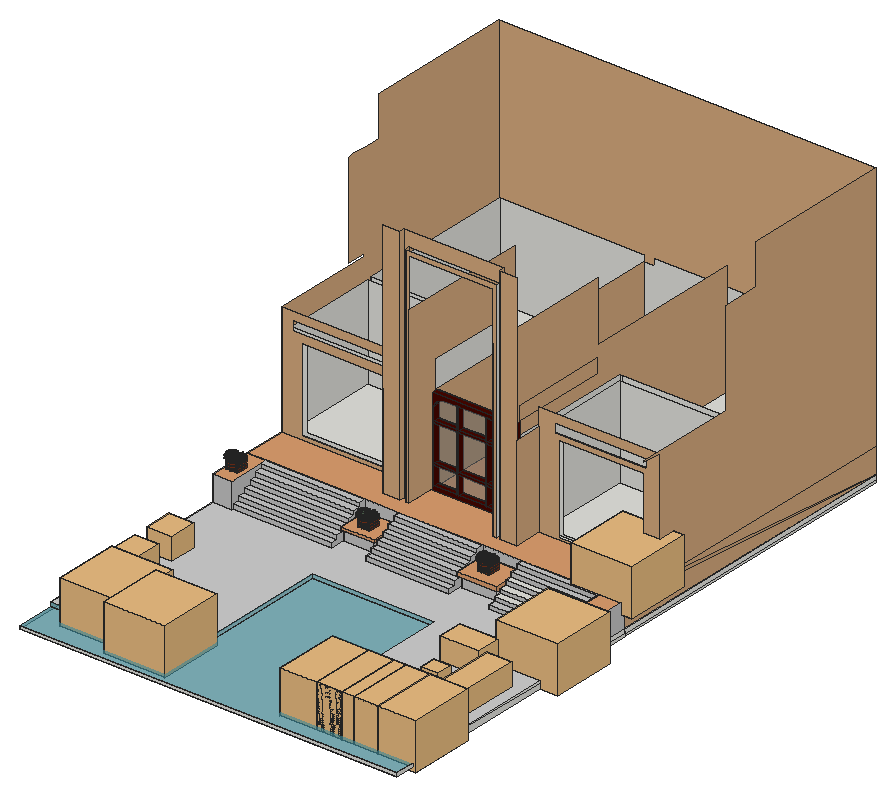
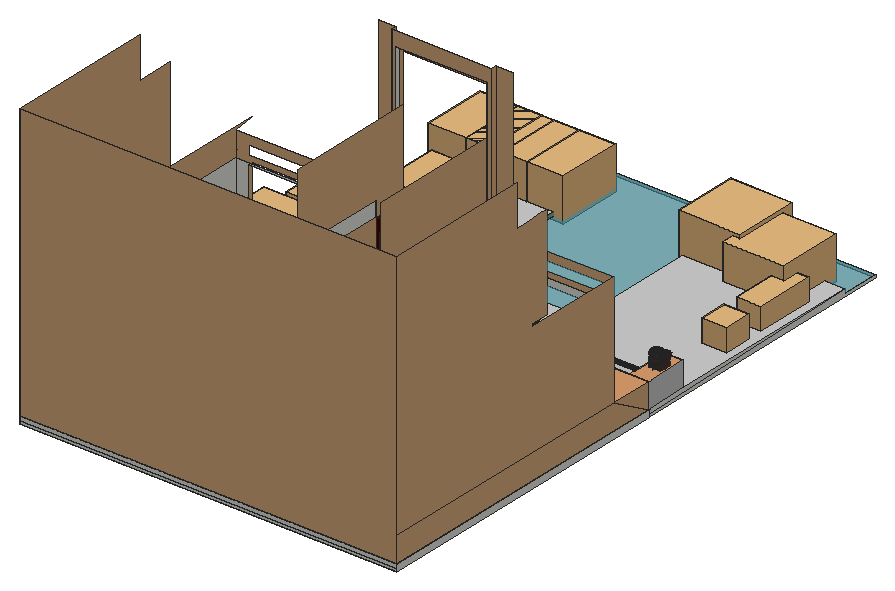
# SketchUp Ruby script. Lengths in inches.
U = 1.inch
M = Sketchup.active_model
def pt(a) = Geom::Point3d.new(a.map { |v| v * U })
def face(e, loops, mat)
  f = e.add_face(loops[0].map { |a| pt(a) })
  loops[1..].each { |l| e.add_face(l.map { |a| pt(a) }).erase! }
  f.material = f.back_material = mat if mat
  f
end
# faces: each face lists its corners as indices into pts; further lists are holes
def faces(e, pts, list, mat = nil) = list.each { |f| face(e, (f[0].is_a?(Array) ? f : [f]).map { |l| l.map { |i| pts[i] } }, mat) }
# xy, xz, yz: faces in a plane at the given z, y or x. An outline is a flat list of corners, or four numbers for a rectangle; further outlines are holes
def ring(l) = l.size == 4 ? [[l[0], l[1]], [l[2], l[1]], [l[2], l[3]], [l[0], l[3]]] : l.each_slice(2).to_a
def flat(e, list, mat, &to3) = list.each { |f| face(e, (f[0].is_a?(Array) ? f : [f]).map { |l| ring(l).map { |u, v| to3.(u, v) } }, mat) }
def xy(e, z, list, mat = nil) = flat(e, list, mat) { |x, y| [x, y, z] }
def xz(e, y, list, mat = nil) = flat(e, list, mat) { |x, z| [x, y, z] }
def yz(e, x, list, mat = nil) = flat(e, list, mat) { |y, z| [x, y, z] }
def lines(e, pts, list) = list.each { |a, b| e.add_line(pt(pts[a]), pt(pts[b])) }
# prism: a flat outline (further loops are holes) pulled along v
def prism(e, loops, v, mat = nil)
  f = face(e, loops, mat); d = Geom::Vector3d.new(v.map { |x| x * U })
  f.pushpull(f.normal.samedirection?(d) ? d.length : -d.length)
end
def box(e, o, s, mat = nil) = prism(e, [[o, [o[0] + s[0], o[1], o[2]], [o[0] + s[0], o[1] + s[1], o[2]], [o[0], o[1] + s[1], o[2]]]], [0, 0, s[2]], mat)
def at(x, y, z, deg = 0) = Geom::Transformation.translation(pt([x, y, z])) * Geom::Transformation.rotation(ORIGIN, Z_AXIS, deg.degrees)
def axes(o, x, y, z) = Geom::Transformation.new([*x, 0, *y, 0, *z, 0, *pt(o).to_a, 1])
def part(name) = M.definitions.add(name)
# library, detail: a bought-in or finely detailed component or shape, given as its bounding box
def library(name, o, s) = part(name).tap { |d| box(d.entities, o, s) }
def detail(e, o, s) = box(e.add_group.entities, o, s)
def put(e, d, t, mat = nil) = e.add_instance(d, t).tap { |i| i.material = mat if mat }
def group(e, t, mat = nil) = e.add_group.tap { |g| g.transformation = t; g.material = mat if mat }.entities
root = M.entities
M.materials.add("24").color = [120, 49, 24]
M.materials.add("[Carrera Marble]").color = [207, 207, 207]
M.materials.add("[Color C04]").color = [215, 171, 127]
M.materials.add("[Color C04]1").color = [220, 158, 110]
M.materials.add("[Color C08]").color = [71, 7, 0]
M.materials.add("[Color M02]").color = [198, 198, 198]
M.materials.add("[Color_G20]").color = [81, 102, 81]
M.materials.add("[Translucent Glass Gray]").color = [128, 128, 128]
M.materials["[Translucent Glass Gray]"].alpha = 0.5
M.materials.add("[Water Pool Light]").color = [64, 149, 167]
M.materials["[Water Pool Light]"].alpha = 0.6
c1 = library("VASO",[-61.49,-57.125,-14.62],[117.55,124.5,88.55])
c2 = library("Group\#4",[0,0,0],[47.0625,53.38,42.38])
c3 = part("3 Leaves\#1")
g1 = group(c3.entities,at(19.98,16.45,10.46))
p = [[9.41,-13.74,-5.37],[9.39,-13.76,-5.36],[9.41,-13.74,-5.375],[-2.22,-4.52,-2],[-1.83,-5.58,-2.64],[-1.27,-6.61,-3.21],
  [-0.57,-7.58,-3.71],[0.27,-8.49,-4.12],[1.23,-9.31,-4.4375],[2.29,-10.02,-4.66],[3.44,-10.62,-4.77],[4.65,-11.09,-4.78],
  [5.91,-11.43,-4.6875],[7.18,-11.625,-4.49],[-2.5,-2.36,-0.58],[-2.44,-3.4375,-1.3125],[0.95,-3.95,0.875],[-0.22,-3.3,0.57],
  [-1.375,-2.77,0.09],[7.11,-10.89,-3.34],[6.85,-10.07,-2.28],[6.41,-9.18,-1.33],[5.81,-8.27,-0.52],[5.05,-7.33,0.125],
  [4.16,-6.41,0.6],[3.16,-5.53,0.89],[2.08,-4.7,0.98],[7.17,-11.64,-4.47],[7.19,-11.61,-4.47]]
faces(g1,p,[[0,1,2],[13,27,28]])
faces(g1,p,[[3,4,5,6,7,8,9,10,11,12,13,14,15],[16,17,18,14,13,19,20,21,22,23,24,25,26]],"[Color_G20]")
g2 = group(c3.entities,at(13.74,14.6,8.97))
p = [[1.36,-2.61,0.95],[2.62,-2.08,0.98],[-2.43,-12.26,-7.12],[-3.0625,-11.53,-6.15],[-3.5,-10.7,-5.16],[-3.74,-9.79,-4.17],
  [-3.77,-8.82,-3.21],[-3.58,-7.83,-2.29],[-3.18,-6.82,-1.46],[-2.59,-5.84,-0.71],[-1.82,-4.91,-0.09],[-0.89,-4.04,0.4],
  [0.18,-3.27,0.75],[-2.43,-12.27,-7.1],[-2.45,-12.25,-7.12],[3.08,-3.14,0.39],[3.37,-4.23,-0.27],[3.49,-5.32,-0.97],
  [3.44,-6.39,-1.7],[3.22,-7.43,-2.45],[2.83,-8.42,-3.21],[2.28,-9.33,-3.96],[1.58,-10.15,-4.68],[0.74,-10.86,-5.375],
  [-0.22,-11.46,-6.02],[-1.28,-11.93,-6.6]]
faces(g2,p,[[0,1,2,3,4,5,6,7,8,9,10,11,12],[2,1,15,16,17,18,19,20,21,22,23,24,25]],"[Color_G20]")
faces(g2,p,[[2,13,14]])
g3 = group(c3.entities,at(16.49,16.82,11.875))
p = [[-2.139,-4.641,-1.793],[-3.318,-5.181,-1.896],[-4.545,-5.609,-1.87],[-5.8,-5.919,-1.717],[-7.057,-6.104,-1.439],[-8.294,-6.16,-1.042],
  [-9.489,-6.087,-0.532],[-10.619,-5.887,0.08],[-11.663,-5.562,0.784],[-12.603,-5.119,1.567],[-13.421,-4.566,2.414],[-0.012,-3.269,-1.214],
  [-1.03,-4,-1.565],[-2.329,-2.745,2.079],[-1.383,-2.856,1.1],[-0.604,-3.033,-0.007],[-12.358,-4.169,3.173],[-11.176,-3.803,3.75],
  [-9.905,-3.478,4.129],[-8.58,-3.2,4.3],[-7.233,-2.979,4.259],[-5.901,-2.82,4.008],[-4.617,-2.726,3.552],[-3.416,-2.701,2.903],
  [-13.414,-4.583,2.432],[-13.418,-4.547,2.431],[-16.492,-4.844,3.262],[-16.488,-4.881,3.264],[-16.492,-4.849,3.258]]
faces(g3,p,[[0,1,2,3,4,5,6,7,8,9,10,11,12],[13,14,15,11,10,16,17,18,19,20,21,22,23]],"[Color_G20]")
faces(g3,p,[[10,24,25],[26,27,28]])
c4 = part("Leaf Array\#1")
put(c4.entities,c3,at(56.94,95.1875,8.9,-157.4))
put(c4.entities,c3,axes([-2.23,49.3,11.63],[0.21933,-0.96954,0.10899],[0.95846,0.19324,-0.20981],[0.18236,0.15048,0.97165]))
put(c4.entities,c3,axes([2.58,75.3,9.0625],[-0.04358,-0.80475,0.59201],[0.73711,-0.51378,-0.32721],[0.78844,0.34173,0.6633]))
put(c4.entities,c3,axes([16.61,3.93,1.625],[0.9836,-0.10453,0.147],[0.10338,0.99452,0.01545],[-0.14781,0,0.98902]))
put(c4.entities,c3,axes([27.18,87.29,10.59],[-0.6021,-0.69264,0.39715],[0.75471,-0.65606,0],[0.26055,0.29973,0.91775]))
put(c4.entities,c3,axes([90.22,57.89,-1.98],[-0.73298,0.58513,0.34694],[-0.62388,-0.78152,0],[0.27114,-0.21645,0.93789]))
put(c4.entities,c3,axes([95.88,23.68,10.66],[-0.09137,0.99511,0.03764],[-0.9603,-0.07804,-0.26784],[-0.26359,-0.06062,0.96273]))
put(c4.entities,c3,axes([45.25,-1.57,4.18],[0.96861,0.19423,0.15515],[-0.19179,0.98096,-0.03072],[-0.15816,0,0.98741]))
put(c4.entities,c3,axes([35.75,0.34,1.875],[0.875,-0.03349,0.48296],[-0.03349,0.99103,0.12941],[-0.48296,-0.12941,0.86603]))
put(c4.entities,c3,axes([66.05,86.7,1.34],[-0.86505,-0.39479,0.30957],[0.40012,-0.91515,-0.04903],[0.30266,0.08145,0.94961]))
put(c4.entities,c3,axes([8.83,45.87,-5.0625],[0.29904,-0.81276,0.5],[0.93849,0.3453,0],[-0.17265,0.46925,0.86603]))
put(c4.entities,c3,axes([7.7,13.9,5.76],[0.75022,-0.49792,0.43502],[0.56511,0.82444,-0.03094],[-0.34324,0.26904,0.89989]))
c5 = part("Hanging Plant 01")
p = [[-9.93,-90.01,162.88],[-9.98,-90.02,162.91],[-10.03,-89.99,162.92],[-10.06,-89.95,162.92],[-10.0625,-89.89,162.91],[-10.03,-89.85,162.88],
  [-9.98,-89.84,162.85],[-9.93,-89.86,162.83],[-9.9,-89.91,162.83],[-9.9,-89.97,162.85]]
faces(c5.entities,p,[[0,1,2,3,4,5,6,7,8,9]])
put(c5.entities,c4,axes([-15.57,-22.79,131.6875],[-0.1651,-0.95585,0],[0.91426,-0.15792,0.07954],[-0.08246,0.01424,0.97612]))
put(c5.entities,c4,axes([64.58,-40.63,128.71],[-0.90863,0.15695,0],[-0.15695,-0.90863,0],[0,0,0.92208]))
put(c5.entities,c4,axes([-7.66,-120.29,132.27],[0.7862,0.27514,0.13834],[-0.29277,0.78542,0.10177],[-0.09553,-0.14273,0.82671]))
put(c5.entities,c4,axes([36.75,-31.84,149.15],[-0.72307,-0.26723,0],[0.26622,-0.72032,-0.06719],[0.02329,-0.06302,0.76794]))
put(c5.entities,c4,axes([13.28,-118.41,149.51],[0.53531,0.55239,0],[-0.54156,0.52481,0],[0,0,0.75413]))
put(c5.entities,c4,axes([19,-32.26,158.75],[-0.44247,-0.37812,0.01283],[0.3708,-0.4339,0],[0.00956,0.00817,0.57062]))
put(c5.entities,c4,axes([-3.99,-97.05,157.98],[0.45934,0.09114,0.05916],[-0.09006,0.45391,0],[-0.07987,-0.01585,0.64455]))
put(c5.entities,c4,axes([-0.45,-92.15,163.74],[0.35828,0.07109,0.04614],[-0.07025,0.35405,0],[-0.0623,-0.01236,0.50275]))
put(c5.entities,c4,axes([1.47,-86.01,171.08],[0.22967,0.04557,0.02958],[-0.04503,0.22696,0],[-0.03993,-0.00792,0.32227]))
c6 = part("Planta de techo redonda")
put(c6.entities,c5,axes([78.49,32.65,14.17],[-0.465,0,0],[0,-0.465,0],[0,0,0.465]))
c7 = part("Group\#84")
box(c7.entities,[0,0,0],[1.57,1.57,15.75])
c8 = part("Group\#85")
put(c8.entities,c7,axes([1.57,0,1.57],[0,0,-1],[0,1,0],[0.825,0,0]),"24")
put(c8.entities,c7,axes([0,12.99,1.57],[0,0,-1],[1,0,0],[0,-0.825,0]),"24")
put(c8.entities,c7,axes([14.57,12.99,1.57],[0,0,-1],[1,0,0],[0,-0.825,0]),"24")
put(c8.entities,c7,axes([1.57,11.42,1.57],[0,0,-1],[0,1,0],[0.825,0,0]),"24")
c9 = part("Group\#86")
put(c9.entities,c8,at(0,11.41,1.57,-45))
put(c9.entities,c8,at(1.78,4.41,0))
c10 = part("FlOwEr BoX")
g4 = group(c10.entities,at(20.46,17.4,0,180))
put(g4,c6,axes([-19.79,-13.06,-13.91],[0.38,0,0],[0,0.38,0],[0,0,0.3306]))
put(g4,c6,axes([-9.47,-13.06,-13.91],[0.38,0,0],[0,0.38,0],[0,0,0.3306]))
put(g4,c9,at(2.54,0,3.15))
put(g4,c9,at(2.54,0,0))
put(g4,c9,at(2.54,0,6.3))
put(g4,c9,at(2.54,0,9.45))
c11 = part("Group\#1")
xy(c11.entities,0,[[0,0,133.1875,11.375]],"[Color C08]")
xy(c11.entities,6.44,[[6.44,0,42.59,11.375],[44.75,0,86.9,11.375],[89.0625,0,126.75,11.375]],"[Color C08]")
xy(c11.entities,37.85,[[6.44,0,42.59,11.375],[44.75,0,86.9,11.375],[89.0625,0,126.75,11.375]],"[Color C08]")
xy(c11.entities,40.75,[[6.44,0,42.59,11.375],[44.75,0,86.9,11.375],[89.0625,0,126.75,11.375]],"[Color C08]")
xy(c11.entities,101.6,[[6.44,0,42.59,11.375],[44.75,0,86.9,11.375],[89.0625,0,126.75,11.375]],"[Color C08]")
xy(c11.entities,104.5,[[6.44,0,42.59,11.375],[44.75,0,86.9,11.375],[89.0625,0,126.75,11.375]],"[Color C08]")
xy(c11.entities,140.62,[[24.51,0,42.59,11.375],[44.75,0,86.9,11.375],[89.0625,0,107.9,11.375]],"[Color C08]")
xy(c11.entities,147.0625,[[0,0,133.1875,11.375]],"[Color C08]")
xz(c11.entities,0,[[[0,0,133.1875,147.0625],[44.75,40.75,86.9,101.6],[89.0625,40.75,126.75,101.6],[6.44,40.75,42.59,101.6],[44.75,104.5,86.9,140.62],[44.75,6.44,86.9,37.85],[89.0625,104.5,89.0625,140.62,107.9,140.62,110.36,140.46,112.78,139.98,115.11,139.1875,117.33,138.1,119.375,136.73,121.23,135.1,122.85,133.25,124.22,131.2,125.3125,128.99,126.1,126.66,126.58,124.24,126.75,121.78,126.75,104.5],[6.44,104.5,6.44,127.03,6.65,127.83,7.8,130.52,9.36,133,11.29,135.21,13.53,137.09,16.03,138.61,18.75,139.72,21.59,140.39,24.51,140.62,42.59,140.62,42.59,104.5],[89.0625,6.44,126.75,37.85],[6.44,6.44,42.59,37.85]]],"[Color C08]")
xz(c11.entities,11.375,[[[0,0,133.1875,147.0625],[44.75,40.75,86.9,101.6],[89.0625,40.75,126.75,101.6],[6.44,40.75,42.59,101.6],[44.75,104.5,86.9,140.62],[44.75,6.44,86.9,37.85],[89.0625,104.5,126.75,104.5,126.75,121.78,126.58,124.24,126.1,126.66,125.3125,128.99,124.22,131.2,122.85,133.25,121.23,135.1,119.375,136.73,117.33,138.1,115.11,139.1875,112.78,139.98,110.36,140.46,107.9,140.62,89.0625,140.62],[6.44,104.5,42.59,104.5,42.59,140.62,24.51,140.62,21.59,140.39,18.75,139.72,16.03,138.61,13.53,137.09,11.29,135.21,9.36,133,7.8,130.52,6.65,127.83,6.44,127.03],[89.0625,6.44,126.75,37.85],[6.44,6.44,42.59,37.85]]],"[Color C08]")
xz(c11.entities,11.375,[[6.44,6.44,42.59,37.85],[44.75,6.44,86.9,37.85],[89.0625,6.44,126.75,37.85],[6.44,40.75,42.59,101.6],[44.75,40.75,86.9,101.6],
  [89.0625,40.75,126.75,101.6],[6.44,104.5,42.59,104.5,42.59,140.62,24.51,140.62,21.59,140.39,18.75,139.72,16.03,138.61,13.53,137.09,11.29,135.21,9.36,133,7.8,130.52,6.65,127.83,6.44,127.03],[44.75,104.5,86.9,140.62],[89.0625,104.5,126.75,104.5,126.75,121.78,126.58,124.24,126.1,126.66,125.3125,128.99,124.22,131.2,122.85,133.25,121.23,135.1,119.375,136.73,117.33,138.1,115.11,139.1875,112.78,139.98,110.36,140.46,107.9,140.62,89.0625,140.62]],"[Translucent Glass Gray]")
yz(c11.entities,0,[[0,0,11.375,147.0625]],"[Color C08]")
yz(c11.entities,6.44,[[0,6.44,11.375,37.85],[0,40.75,11.375,101.6],[0,104.5,11.375,127.03]],"[Color C08]")
yz(c11.entities,42.59,[[0,6.44,11.375,37.85],[0,40.75,11.375,101.6],[0,104.5,11.375,140.62]],"[Color C08]")
yz(c11.entities,44.75,[[0,6.44,11.375,37.85],[0,40.75,11.375,101.6],[0,104.5,11.375,140.62]],"[Color C08]")
yz(c11.entities,86.9,[[0,6.44,11.375,37.85],[0,40.75,11.375,101.6],[0,104.5,11.375,140.62]],"[Color C08]")
yz(c11.entities,89.0625,[[0,6.44,11.375,37.85],[0,40.75,11.375,101.6],[0,104.5,11.375,140.62]],"[Color C08]")
yz(c11.entities,126.75,[[0,6.44,11.375,37.85],[0,40.75,11.375,101.6],[0,104.5,11.375,121.78]],"[Color C08]")
yz(c11.entities,133.1875,[[0,0,11.375,147.0625]],"[Color C08]")
p = [[126.58,11.375,124.24],[126.75,11.375,121.78],[126.75,0,121.78],[126.58,0,124.24],[126.1,11.375,126.66],[126.1,0,126.66],
  [125.3125,11.375,128.99],[125.3125,0,128.99],[6.44,11.375,127.03],[6.65,11.375,127.83],[6.65,0,127.83],[6.44,0,127.03],
  [7.8,11.375,130.52],[7.8,0,130.52],[124.22,11.375,131.2],[124.22,0,131.2],[9.36,11.375,133],[9.36,0,133],
  [122.85,11.375,133.25],[122.85,0,133.25],[11.29,11.375,135.21],[11.29,0,135.21],[121.23,11.375,135.1],[121.23,0,135.1],
  [119.375,11.375,136.73],[119.375,0,136.73],[13.53,11.375,137.09],[13.53,0,137.09],[117.33,11.375,138.1],[117.33,0,138.1],
  [16.03,11.375,138.61],[16.03,0,138.61],[115.11,11.375,139.1875],[115.11,0,139.1875],[18.75,11.375,139.72],[18.75,0,139.72],
  [112.78,11.375,139.98],[112.78,0,139.98],[21.59,11.375,140.39],[21.59,0,140.39],[110.36,11.375,140.46],[110.36,0,140.46],
  [24.51,11.375,140.62],[24.51,0,140.62],[107.9,11.375,140.62],[107.9,0,140.62]]
faces(c11.entities,p,[[0,1,2,3],[4,0,3,5],[6,4,5,7],[8,9,10,11],[9,12,13,10],[14,6,7,15],[12,16,17,13],[18,14,15,19],
  [16,20,21,17],[22,18,19,23],[24,22,23,25],[20,26,27,21],[28,24,25,29],[26,30,31,27],[32,28,29,33],[30,34,35,31],
  [36,32,33,37],[34,38,39,35],[40,36,37,41],[38,42,43,39],[44,40,41,45]],"[Color C08]")
xy(root,-4.9375,[[19.375,0,739.375,543.4375],[18.75,543.4375,738.75,1143.4375]])
xy(root,0.5625,[[19.375,0,739.375,0,739.375,72.86,504.4375,72.86,504.4375,383.55,271.8125,383.55,271.8125,72.86,19.375,72.86]],"[Water Pool Light]")
xy(root,9,[[18.75,460.5625,18.86,460.5625,18.75,543.4375],[18.86,460.5625,18.75,543.4375,54.9375,543.4375,54.9375,460.5625],[54.9375,463.52,244.08,476.84],[309.07,463.52,467.95,476.84],[544.14,463.52,698.27,476.84],
  [698.27,465.72,698.27,543.4375,738.75,543.4375,738.85,465.72],[738.85,465.72,738.85,543.4375,738.75,543.4375],[54.9375,476.84,244.08,543.4375],[309.07,476.84,467.95,543.4375],[544.14,476.84,698.27,543.4375],
  [18.75,543.4375,738.75,1143.4375]])
xy(root,9,[[19.375,72.86,271.8125,72.86,271.8125,383.55,504.4375,383.55,504.4375,72.86,739.375,72.86,738.85,465.72,698.27,465.72,698.27,463.52,544.14,463.52,544.14,543.4375,537.39,543.4375,538.02,490.125,471.39,490.125,470.77,543.4375,467.95,543.4375,467.95,463.52,309.07,463.52,309.07,543.4375,302.77,543.4375,303.39,490.125,246.52,490.125,245.89,543.4375,244.08,543.4375,244.08,463.52,54.9375,463.52,54.9375,460.5625,18.86,460.5625]],"[Carrera Marble]")
xy(root,17,[[54.9375,463.52,244.08,476.84],[309.07,463.52,467.95,476.84],[544.14,463.52,698.27,476.84]],"[Color M02]")
xy(root,25,[[544.14,476.84,698.27,490.16]])
xy(root,25,[[54.9375,476.84,244.08,490.16],[309.07,476.84,467.95,490.16]],"[Color M02]")
xy(root,30.4375,[[244.7,485.3125,244.08,543.4375,245.89,543.4375,246.52,490.125,303.39,490.125,302.77,543.4375,308.45,543.4375,309.08,485.3125]])
xy(root,31.0625,[[468.58,482.375,467.95,543.4375,470.77,543.4375,471.39,490.125,538.02,490.125,537.39,543.4375,543.52,543.4375,544.14,482.375]])
xy(root,31.9375,[[246.52,490.125,303.39,543.4375]])
xy(root,32.6875,[[471.39,490.125,538.02,543.4375]])
xy(root,33,[[544.14,490.16,698.27,503.48]])
xy(root,33,[[54.9375,490.16,244.08,503.48],[309.07,490.16,467.95,503.48]],"[Color M02]")
xy(root,35.9375,[[244.7,485.3125,309.08,485.3125,308.45,543.4375,244.08,543.4375]],"[Color C04]1")
xy(root,38.5625,[[468.58,482.375,544.14,482.375,543.52,543.4375,467.95,543.4375]],"[Color C04]1")
xy(root,41,[[544.14,503.48,698.27,516.8]])
xy(root,41,[[54.9375,503.48,244.08,516.8],[309.07,503.48,467.95,516.8]],"[Color M02]")
xy(root,49,[[54.9375,516.8,244.08,530.12],[309.07,516.8,467.95,530.12],[544.14,516.8,698.27,530.12]],"[Color M02]")
xy(root,57,[[258.9375,590.9375,303.29,590.9375,303.29,1134.4375,28.375,1134.4375,28.375,826.1875,258.9375,826.1875],[462.79,590.9375,503.3125,590.9375,503.3125,826.375,509.3125,826.1875,730.375,826.1875,730.375,1134.4375,462.79,1134.4375],[28.375,638.0625,252.9375,820.1875],[509.3125,638.0625,730.375,820.1875]])
xy(root,57,[[18.86,460.5625,54.9375,460.5625,54.9375,543.4375,18.75,543.4375],[698.27,465.72,738.85,465.72,738.75,543.4375,698.27,543.4375],[18.75,543.4375,19.375,626.0625,252.9375,626.0625,252.9375,573.625,285.62,573.625,285.62,583.375,296.34,583.375,296.34,574.1875,303.29,574.1875,303.29,1134.4375,462.79,1134.4375,462.79,574.1875,470.03,574.1875,470.03,583.375,477.47,583.375,477.47,573.625,509.3125,573.625,509.3125,627.4375,739.375,627.4375,738.75,543.4375]],"[Color C04]1")
xy(root,57,[[54.9375,530.12,244.08,543.4375],[309.07,530.12,467.95,543.4375],[544.14,530.12,698.27,543.4375]],"[Color M02]")
xz(root,0,[[19.375,-4.9375,739.375,0.5625]])
xz(root,72.86,[[19.375,0.5625,271.8125,9],[504.4375,0.5625,739.375,9]],"[Water Pool Light]")
xz(root,383.55,[[271.8125,0.5625,504.4375,9]],"[Water Pool Light]")
xz(root,460.5625,[[18.86,9,54.9375,57]],"[Color M02]")
xz(root,463.52,[[54.9375,9,244.08,17],[309.07,9,467.95,17],[544.14,9,698.27,17]],"[Color M02]")
xz(root,465.72,[[698.27,9,738.85,57]],"[Color M02]")
xz(root,476.84,[[54.9375,17,244.08,25],[309.07,17,467.95,25],[544.14,17,698.27,25]],"[Color M02]")
xz(root,482.375,[[468.58,31.0625,544.14,38.5625]],"[Color C04]1")
xz(root,485.3125,[[244.7,30.4375,309.08,35.9375]],"[Color C04]1")
xz(root,490.125,[[246.52,30.4375,303.39,31.9375],[471.39,31.0625,538.02,32.6875]])
xz(root,490.125,[[246.52,9,303.39,30.4375],[471.39,9,538.02,31.0625]],"[Color M02]")
xz(root,490.16,[[54.9375,25,244.08,33],[309.07,25,467.95,33],[544.14,25,698.27,33]],"[Color M02]")
xz(root,503.48,[[54.9375,33,244.08,41],[309.07,33,467.95,41],[544.14,33,698.27,41]],"[Color M02]")
xz(root,516.8,[[54.9375,41,244.08,49],[309.07,41,467.95,49],[544.14,41,698.27,49]],"[Color M02]")
xz(root,530.12,[[54.9375,49,244.08,57],[309.07,49,467.95,57],[544.14,49,698.27,57]],"[Color M02]")
xz(root,543.4375,[[18.75,-4.9375,19.375,-4.9375,19.375,0,18.75,9],[19.375,-4.9375,19.375,0,18.75,9,54.9375,9,54.9375,-4.9375],[54.9375,-4.9375,244.08,9],[244.08,-4.9375,245.89,9],[245.89,-4.9375,302.77,9],
  [302.77,-4.9375,309.07,9],[309.07,-4.9375,467.95,9],[467.95,-4.9375,470.77,9],[470.77,-4.9375,537.39,9],[537.39,-4.9375,544.14,9],
  [544.14,-4.9375,698.27,9],[698.27,-4.9375,738.75,9],[738.75,-4.9375,738.75,9,739.375,0,739.375,-4.9375],[18.75,9,54.9375,57],[54.9375,9,244.08,49],
  [244.08,9,245.89,30.4375],[245.89,9,302.77,9,302.77,30.4375,303.39,31.9375,246.52,31.9375,245.89,30.4375],[309.07,9,467.95,49],[467.95,9,470.77,31.0625],[470.77,9,537.39,9,537.39,31.0625,538.02,32.6875,471.39,32.6875,470.77,31.0625],
  [544.14,9,698.27,49],[698.27,9,738.75,57],[244.08,30.4375,245.89,30.4375,246.52,31.9375,303.39,31.9375,302.77,30.4375,308.45,30.4375,308.45,35.9375,244.08,35.9375],[467.95,31.0625,470.77,31.0625,471.39,32.6875,538.02,32.6875,537.39,31.0625,543.52,31.0625,543.52,38.5625,467.95,38.5625],[54.9375,49,244.08,57],
  [309.07,49,467.95,57],[544.14,49,698.27,57]])
xz(root,543.4375,[[302.77,9,309.07,9,309.07,57,244.08,57,244.08,35.9375,308.45,35.9375,308.45,30.4375,302.77,30.4375],[537.39,9,544.14,9,544.14,57,467.95,57,467.95,38.5625,543.52,38.5625,543.52,31.0625,537.39,31.0625]],"[Color M02]")
xz(root,573.625,[[252.9375,57,285.62,516.1875],[477.47,57,509.3125,516.1875]],"[Color C04]")
xz(root,574.1875,[[296.34,57,303.29,57,303.29,480.375,462.79,480.375,462.79,57,470.03,57,470.03,489.0625,296.34,489.0625]],"[Color C04]")
xz(root,583.375,[[285.62,57,296.34,57,296.34,489.0625,470.03,489.0625,470.03,57,477.47,57,477.47,516.1875,285.62,516.1875]],"[Color C04]")
xz(root,626.0625,[[[19.375,57,252.9375,271.1875],[57.38,63.5625,219.82,221.625],[40.76,237,228.51,255.5]]],"[Color C04]")
xz(root,627.4375,[[[509.3125,57,739.375,57,739.375,237,539.72,237,539.72,254.125,714.84,254.125,714.84,237,739.375,237,739.375,271.1875,509.3125,271.1875],[546.77,60.79,708.59,227.85]]],"[Color C04]")
xz(root,638.0625,[[[28.375,57,252.9375,235],[57.38,63.5625,219.82,221.625]],[[509.3125,57,730.375,231],[546.77,60.79,708.59,227.85]]])
xz(root,820.1875,[[28.375,57,252.9375,235],[509.3125,57,730.375,231]])
xz(root,826.1875,[[28.375,57,258.9375,237],[509.3125,57,730.375,237]])
xz(root,1134.4375,[[28.375,57,303.29,237],[303.29,57,462.79,57,462.79,237,323.73,237,323.73,224.25,303.29,224.25],[462.79,57,730.375,237]])
xz(root,1143.4375,[[18.75,-4.9375,18.75,9,19.375,0,738.75,0,738.75,-4.9375],[19.375,0,18.75,9,738.75,9,738.75,0],[738.75,0,738.75,9,739.375,0]])
xz(root,1143.4375,[[18.75,9,19.375,57,19.375,533.8125,739.375,533.8125,739.375,57,738.75,9]],"[Color C04]")
yz(root,18.75,[[543.4375,-4.9375,1143.4375,9]])
yz(root,19.375,[[0,-4.9375,0,0.5625,72.86,0.5625,72.86,9,543.4375,0,543.4375,-4.9375]])
yz(root,19.375,[[626.0625,57,626.0625,271.1875,820.1875,271.1875,820.1875,276.1875,784.25,276.1875,784.25,456.1875,798.1875,458.3,826.1875,456.1875,857.1875,456.1875,857.1875,533.8125,1143.4375,533.8125,1143.4375,57]],"[Color C04]")
yz(root,28.375,[[638.0625,57,820.1875,235],[826.1875,57,1134.4375,237]])
yz(root,54.9375,[[460.5625,9,463.52,9,463.52,17,476.84,17,476.84,25,490.16,25,490.16,33,503.48,33,503.48,41,516.8,41,516.8,49,530.12,49,530.12,57,460.5625,57]],"[Color M02]")
yz(root,244.08,[[463.52,9,543.4375,9,543.4375,57,530.12,57,530.12,49,516.8,49,516.8,41,503.48,41,503.48,33,490.16,33,490.16,25,476.84,25,476.84,17,463.52,17]],"[Color M02]")
yz(root,246.52,[[490.125,30.4375,490.125,31.9375,543.4375,31.9375]])
yz(root,252.9375,[[638.0625,57,820.1875,235]])
yz(root,252.9375,[[573.625,57,626.0625,237]],"[Color C04]")
yz(root,258.9375,[[590.9375,57,826.1875,237]])
yz(root,271.8125,[[72.86,0.5625,383.55,9]],"[Water Pool Light]")
yz(root,285.62,[[573.625,57,583.375,516.1875]],"[Color C04]")
yz(root,296.34,[[574.1875,57,583.375,489.0625]],"[Color C04]")
yz(root,303.29,[[574.1875,57,1134.4375,57,1134.4375,224.25,636.875,224.25,636.875,276.1875,826.22,276.1875,826.22,387.35,574.1875,387.35]],"[Color C04]")
yz(root,309.07,[[463.52,9,463.52,17,476.84,17,476.84,25,490.16,25,490.16,33,503.48,33,503.48,41,516.8,41,516.8,49,530.12,49,530.12,57,543.4375,57,543.4375,9]],"[Color M02]")
yz(root,462.79,[[574.1875,57,574.1875,387.35,826.22,387.35,826.22,276.1875,826.34,276.1875,826.34,273.1875,1134.4375,273.1875,1134.4375,237,826.22,237,826.22,252.9375,636.875,252.9375,636.875,224.25,826.22,224.25,826.22,237,1134.4375,237,1134.4375,57]],"[Color C04]")
yz(root,467.95,[[463.52,9,543.4375,9,543.4375,57,530.12,57,530.12,49,516.8,49,516.8,41,503.48,41,503.48,33,490.16,33,490.16,25,476.84,25,476.84,17,463.52,17]],"[Color M02]")
yz(root,470.03,[[574.1875,57,583.375,489.0625]])
yz(root,471.39,[[490.125,31.0625,490.125,32.6875,543.4375,32.6875]])
yz(root,477.47,[[573.625,57,583.375,516.1875]],"[Color C04]")
yz(root,503.3125,[[590.9375,57,826.375,237]])
yz(root,504.4375,[[72.86,0.5625,383.55,9]],"[Water Pool Light]")
yz(root,509.3125,[[638.0625,57,820.1875,231]])
yz(root,509.3125,[[573.625,57,627.4375,237]],"[Color C04]")
yz(root,544.14,[[463.52,9,463.52,17,476.84,17,476.84,25,490.16,25,490.16,33,503.48,33,503.48,41,516.8,41,516.8,49,530.12,49,530.12,57,543.4375,57,543.4375,9]],"[Color M02]")
yz(root,698.27,[[463.52,9,465.72,17],[465.72,9,465.72,17,476.84,17,476.84,25,490.16,25,490.16,33,503.48,33,503.48,41,516.8,41,516.8,49,530.12,49,530.12,57,543.4375,57,543.4375,9]])
yz(root,698.27,[[465.72,17,465.72,57,530.12,57,530.12,49,516.8,49,516.8,41,503.48,41,503.48,33,490.16,33,490.16,25,476.84,25,476.84,17]],"[Color M02]")
yz(root,730.375,[[638.0625,57,820.1875,231],[826.1875,57,1134.4375,237]])
yz(root,738.75,[[543.4375,-4.9375,1143.4375,9]])
yz(root,738.75,[[543.4375,9,1143.4375,9,543.4375,57]],"[Color C04]")
yz(root,739.375,[[0,-4.9375,543.4375,-4.9375,543.4375,0,72.86,9,72.86,0.5625,0,0.5625]])
yz(root,739.375,[[627.4375,57,1143.4375,57,1143.4375,533.8125,857.1875,533.8125,857.1875,456.1875,784.25,456.1875,784.25,276.1875,588.625,276.1875,588.625,275.59,627.4375,271.1875]],"[Color C04]")
p = [[18.75,543.4375,9],[19.375,543.4375,0],[19.375,72.86,9],[18.86,460.5625,9],[738.75,543.4375,9],[738.85,465.72,9],
  [739.375,72.86,9],[739.375,543.4375,0],[18.75,1143.4375,9],[19.375,1143.4375,0],[739.375,1143.4375,0],[738.75,1143.4375,9],
  [18.86,460.5625,57],[18.75,543.4375,57],[738.75,543.4375,57],[738.85,465.72,57],[246.52,490.125,30.4375],[245.89,543.4375,30.4375],
  [245.89,543.4375,9],[246.52,490.125,9],[303.39,490.125,9],[302.77,543.4375,9],[302.77,543.4375,30.4375],[303.39,490.125,30.4375],
  [471.39,490.125,31.0625],[470.77,543.4375,31.0625],[470.77,543.4375,9],[471.39,490.125,9],[538.02,490.125,9],[537.39,543.4375,9],
  [537.39,543.4375,31.0625],[538.02,490.125,31.0625],[19.375,626.0625,57],[19.375,1143.4375,57],[739.375,627.4375,57],[739.375,1143.4375,57],
  [244.7,485.3125,35.9375],[244.08,543.4375,35.9375],[244.08,543.4375,30.4375],[244.7,485.3125,30.4375],[309.08,485.3125,30.4375],[308.45,543.4375,30.4375],
  [308.45,543.4375,35.9375],[309.08,485.3125,35.9375],[246.52,543.4375,31.9375],[303.39,490.125,31.9375],[303.39,543.4375,31.9375],[468.58,482.375,38.5625],
  [467.95,543.4375,38.5625],[467.95,543.4375,31.0625],[468.58,482.375,31.0625],[544.14,482.375,31.0625],[543.52,543.4375,31.0625],[543.52,543.4375,38.5625],
  [544.14,482.375,38.5625],[471.39,543.4375,32.6875],[538.02,490.125,32.6875],[538.02,543.4375,32.6875],[509.3125,826.1875,57],[503.3125,826.375,57],
  [503.3125,826.375,237],[509.3125,826.1875,237],[312,490.16,17],[424.94,490.16,17],[312,516.8,33],[424.94,516.8,33],
  [312,530.12,41],[424.94,530.12,41],[89.69,490.16,17],[202.63,490.16,17],[89.69,503.48,25],[202.63,503.48,25],
  [89.69,516.8,33],[202.63,516.8,33],[89.69,530.12,41],[202.63,530.12,41],[678.75,530.12,41],[565.82,530.12,41],
  [678.75,516.8,33],[565.82,516.8,33],[678.75,503.48,25],[565.82,503.48,25],[678.75,490.16,17],[565.82,490.16,17]]
faces(root,p,[[0,1,2,3],[4,5,6,7],[0,8,9,1],[7,10,11,4],[24,25,26,27],[28,29,30,31],[17,16,44],[23,22,45],
  [46,45,22],[25,24,55],[31,30,56],[57,56,30],[58,59,60,61]])
faces(root,p,[[0,3,12,13],[5,4,14,15],[16,17,18,19],[20,21,22,23]],"[Color M02]")
faces(root,p,[[0,32,33,8],[13,32,0],[34,14,11],[35,34,11]],"[Color C04]")
faces(root,p,[[36,37,38,39],[40,41,42,43],[47,48,49,50],[51,52,53,54]],"[Color C04]1")
lines(root,p,[[62,63],[64,65],[66,67],[68,69],[70,71],[72,73],[74,75],[76,77],[78,79],[80,81],[82,83]])
put(root,c1,at(617.59,94.31,2.3125))
put(root,c1,at(688.97,94.31,2.3125))
put(root,c1,at(548.41,94.31,2.3125))
put(root,c1,at(121.07,101.7,2.71))
put(root,c1,at(224.375,77.33,9))
put(root,c1,at(716.4,399.48,9))
put(root,c2,at(36.47,282,9))
put(root,c2,axes([36.47,138.8,9],[1,0,0],[0,2.13,0],[0,0,1]))
put(root,c2,axes([717.97,301.25,9],[-1,0,0],[0,-2.13,0],[0,0,1]))
put(root,c2,axes([666.1,148.85,9],[0,1,0],[-1.38706,0,0],[0,0,1]))
put(root,c2,axes([584.46,343.52,9],[0,-1,0],[1.38706,0,0],[0,0,1]))
g5 = group(root,at(602.72,228.72,9))
detail(g5,[0,0,0],[32.6,30.22,25.56])
put(root,c10,axes([264.375,500.5,35.9375],[1.4022,0,0],[0,1.6851,0],[0,0,1.5029]))
put(root,c1,at(704.28,592.28,52.1875))
put(root,c10,axes([490.16,504.21,38.5625],[1.4022,0,0],[0,1.6851,0],[0,0,1.5029]))
put(root,c10,axes([24.27,486.01,57],[1.4022,0,0],[0,1.6851,0],[0,0,1.5029]))
put(root,c11,axes([299.77,628.36,57],[1.224,0,0],[0,1,0],[0,0,1.136]))
